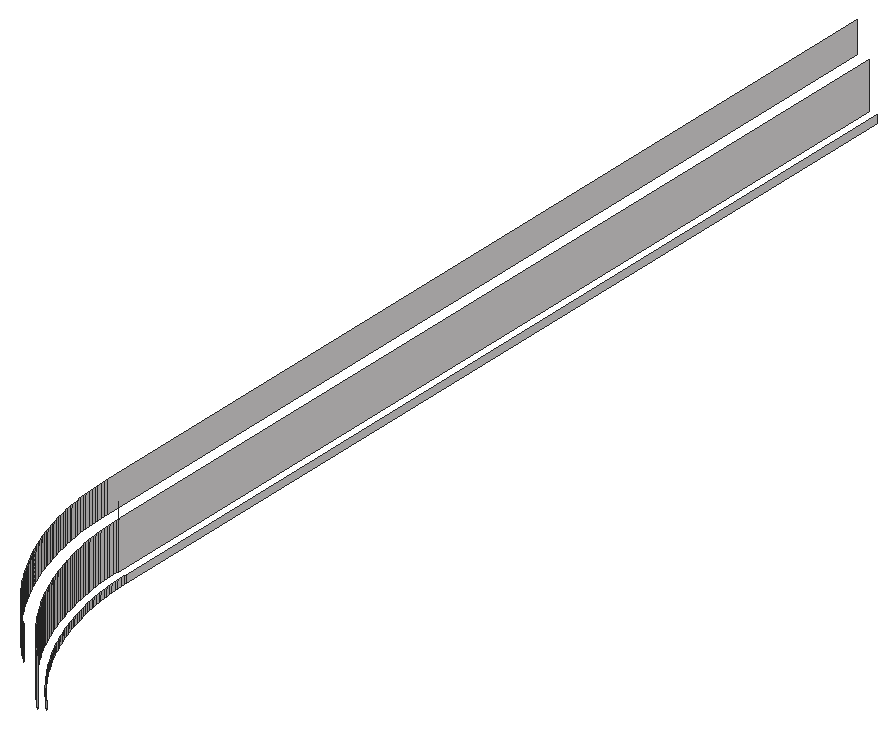
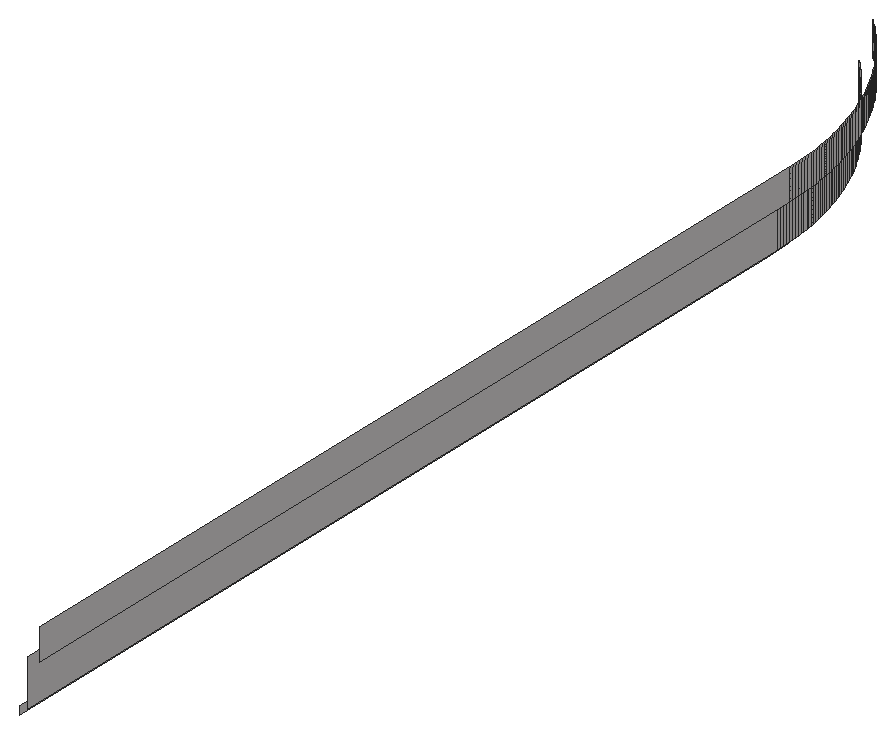
# SketchUp Ruby script. Lengths in inches.
U = 1.inch
M = Sketchup.active_model
def pt(a) = Geom::Point3d.new(a.map { |v| v * U })
def face(e, loops, mat)
  f = e.add_face(loops[0].map { |a| pt(a) })
  loops[1..].each { |l| e.add_face(l.map { |a| pt(a) }).erase! }
  f.material = f.back_material = mat if mat
  f
end
# faces: each face lists its corners as indices into pts; further lists are holes
def faces(e, pts, list, mat = nil) = list.each { |f| face(e, (f[0].is_a?(Array) ? f : [f]).map { |l| l.map { |i| pts[i] } }, mat) }
# xy, xz, yz: faces in a plane at the given z, y or x. An outline is a flat list of corners, or four numbers for a rectangle; further outlines are holes
def ring(l) = l.size == 4 ? [[l[0], l[1]], [l[2], l[1]], [l[2], l[3]], [l[0], l[3]]] : l.each_slice(2).to_a
def flat(e, list, mat, &to3) = list.each { |f| face(e, (f[0].is_a?(Array) ? f : [f]).map { |l| ring(l).map { |u, v| to3.(u, v) } }, mat) }
def xy(e, z, list, mat = nil) = flat(e, list, mat) { |x, y| [x, y, z] }
def xz(e, y, list, mat = nil) = flat(e, list, mat) { |x, z| [x, y, z] }
def yz(e, x, list, mat = nil) = flat(e, list, mat) { |y, z| [x, y, z] }
def lines(e, pts, list) = list.each { |a, b| e.add_line(pt(pts[a]), pt(pts[b])) }
# prism: a flat outline (further loops are holes) pulled along v
def prism(e, loops, v, mat = nil)
  f = face(e, loops, mat); d = Geom::Vector3d.new(v.map { |x| x * U })
  f.pushpull(f.normal.samedirection?(d) ? d.length : -d.length)
end
def box(e, o, s, mat = nil) = prism(e, [[o, [o[0] + s[0], o[1], o[2]], [o[0] + s[0], o[1] + s[1], o[2]], [o[0], o[1] + s[1], o[2]]]], [0, 0, s[2]], mat)
def at(x, y, z, deg = 0) = Geom::Transformation.translation(pt([x, y, z])) * Geom::Transformation.rotation(ORIGIN, Z_AXIS, deg.degrees)
def axes(o, x, y, z) = Geom::Transformation.new([*x, 0, *y, 0, *z, 0, *pt(o).to_a, 1])
def part(name) = M.definitions.add(name)
# library, detail: a bought-in or finely detailed component or shape, given as its bounding box
def library(name, o, s) = part(name).tap { |d| box(d.entities, o, s) }
def detail(e, o, s) = box(e.add_group.entities, o, s)
def put(e, d, t, mat = nil) = e.add_instance(d, t).tap { |i| i.material = mat if mat }
def group(e, t, mat = nil) = e.add_group.tap { |g| g.transformation = t; g.material = mat if mat }.entities
root = M.entities
M.materials.add("[Quartz Light Brown]").color = [215, 212, 212]
yz(root,185.5,[[320.18,493,320.7,497],[320.7,493,440.7,497]],"[Quartz Light Brown]")
yz(root,187,[[320.2,487,320.7,493],[320.7,487,440.7,493]],"[Quartz Light Brown]")
yz(root,188,[[320.22,486,320.7,487],[320.7,486,440.7,487]],"[Quartz Light Brown]")
p = [[197.5,295.94,486],[197.83,295.59,486],[197.83,295.59,487],[197.5,295.94,487],[197.18,296.31,486],[197.18,296.31,487],
  [196.86,296.67,486],[196.86,296.67,487],[196.55,297.04,486],[196.55,297.04,487],[196.25,297.42,486],[196.25,297.42,487],
  [195.94,297.79,486],[195.94,297.79,487],[195.65,298.18,486],[195.65,298.18,487],[195.35,298.5625,486],[195.35,298.5625,487],
  [195.07,298.95,486],[195.07,298.95,487],[194.78,299.35,486],[194.78,299.35,487],[194.51,299.74,486],[194.51,299.74,487],
  [194.24,300.14,486],[194.24,300.14,487],[193.97,300.55,486],[193.97,300.55,487],[193.71,300.96,486],[193.71,300.96,487],
  [193.45,301.37,486],[193.45,301.37,487],[193.2,301.78,486],[193.2,301.78,487],[192.96,302.2,486],[192.96,302.2,487],
  [192.72,302.62,486],[192.72,302.62,487],[192.48,303.05,486],[192.48,303.05,487],[192.26,303.47,486],[192.26,303.47,487],
  [192.03,303.9,486],[192.03,303.9,487],[191.82,304.34,486],[191.82,304.34,487],[191.6,304.77,486],[191.6,304.77,487],
  [191.4,305.21,486],[191.4,305.21,487],[191.2,305.65,486],[191.2,305.65,487],[191,306.1,486],[191,306.1,487],
  [190.82,306.54,486],[190.82,306.54,487],[190.63,306.99,486],[190.63,306.99,487],[190.46,307.44,486],[190.46,307.44,487],
  [190.29,307.89,486],[190.29,307.89,487],[190.12,308.35,486],[190.12,308.35,487],[189.96,308.81,486],[189.96,308.81,487],
  [189.8125,309.27,486],[189.8125,309.27,487],[189.66,309.73,486],[189.66,309.73,487],[189.52,310.19,486],[189.52,310.19,487],
  [189.39,310.66,486],[189.39,310.66,487],[189.26,311.125,486],[189.26,311.125,487],[189.14,311.59,486],[189.14,311.59,487],
  [189.02,312.0625,486],[189.02,312.0625,487],[188.91,312.54,486],[188.91,312.54,487],[188.81,313.01,486],[188.81,313.01,487],
  [188.71,313.48,486],[188.71,313.48,487],[188.62,313.96,486],[188.62,313.96,487],[188.53,314.44,486],[188.53,314.44,487],
  [188.46,314.91,486],[188.46,314.91,487],[188.38,315.39,486],[188.38,315.39,487],[188.32,315.87,486],[188.32,315.87,487],
  [188.26,316.35,486],[188.26,316.35,487],[188.2,316.83,486],[188.2,316.83,487],[188.16,317.32,486],[188.16,317.32,487],
  [188.11,317.8,486],[188.11,317.8,487],[188.08,318.28,486],[188.08,318.28,487],[188.05,318.76,486],[188.05,318.76,487],
  [188.03,319.25,486],[188.03,319.25,487],[188.01,319.73,486],[188.01,319.73,487],[188,320.22,486],[188,320.22,487],
  [198.13,293.83,487],[198.13,293.83,493],[197.78,294.18,493],[197.78,294.18,487],[197.4375,294.54,493],[197.4375,294.54,487],
  [197.1,294.91,493],[197.1,294.91,487],[196.76,295.27,493],[196.76,295.27,487],[196.43,295.65,493],[196.43,295.65,487],
  [196.1,296.02,493],[196.1,296.02,487],[195.78,296.4,493],[195.78,296.4,487],[195.47,296.79,493],[195.47,296.79,487],
  [195.16,297.18,493],[195.16,297.18,487],[194.85,297.57,493],[194.85,297.57,487],[194.55,297.96,493],[194.55,297.96,487],
  [194.26,298.37,493],[194.26,298.37,487],[193.97,298.77,493],[193.97,298.77,487],[193.68,299.18,493],[193.68,299.18,487],
  [193.4,299.59,493],[193.4,299.59,487],[193.13,300,493],[193.13,300,487],[192.86,300.42,493],[192.86,300.42,487],
  [192.6,300.85,493],[192.6,300.85,487],[192.34,301.27,493],[192.34,301.27,487],[192.09,301.7,493],[192.09,301.7,487],
  [191.85,302.13,493],[191.85,302.13,487],[191.6,302.57,493],[191.6,302.57,487],[191.37,303.01,493],[191.37,303.01,487],
  [191.14,303.45,493],[191.14,303.45,487],[190.92,303.89,493],[190.92,303.89,487],[190.7,304.34,493],[190.7,304.34,487],
  [190.49,304.79,493],[190.49,304.79,487],[190.29,305.25,493],[190.29,305.25,487],[190.09,305.7,493],[190.09,305.7,487],
  [189.89,306.16,493],[189.89,306.16,487],[189.71,306.62,493],[189.71,306.62,487],[189.52,307.08,493],[189.52,307.08,487],
  [189.35,307.55,493],[189.35,307.55,487],[189.18,308.02,493],[189.18,308.02,487],[189.02,308.49,493],[189.02,308.49,487],
  [188.86,308.96,493],[188.86,308.96,487],[188.71,309.43,493],[188.71,309.43,487],[188.56,309.91,493],[188.56,309.91,487],
  [188.43,310.39,493],[188.43,310.39,487],[188.29,310.87,493],[188.29,310.87,487],[188.17,311.35,493],[188.17,311.35,487],
  [188.05,311.83,493],[188.05,311.83,487],[187.9375,312.31,493],[187.9375,312.31,487],[187.83,312.8,493],[187.83,312.8,487],
  [187.73,313.29,493],[187.73,313.29,487],[187.64,313.78,493],[187.64,313.78,487],[187.55,314.27,493],[187.55,314.27,487],
  [187.47,314.76,493],[187.47,314.76,487],[187.39,315.25,493],[187.39,315.25,487],[187.33,315.74,493],[187.33,315.74,487],
  [187.26,316.23,493],[187.26,316.23,487],[187.21,316.73,493],[187.21,316.73,487],[187.16,317.22,493],[187.16,317.22,487],
  [187.12,317.72,493],[187.12,317.72,487],[187.08,318.22,493],[187.08,318.22,487],[187.05,318.71,493],[187.05,318.71,487],
  [187.03,319.21,493],[187.03,319.21,487],[187.01,319.71,493],[187.01,319.71,487],[187,320.2,493],[187,320.2,487],
  [197.4375,292.41,493],[197.81,292.05,493],[197.81,292.05,497],[197.4375,292.41,497],[197.07,292.77,493],[197.07,292.77,497],
  [196.71,293.14,493],[196.71,293.14,497],[196.35,293.51,493],[196.35,293.51,497],[195.99,293.89,493],[195.99,293.89,497],
  [195.65,294.27,493],[195.65,294.27,497],[195.3,294.66,493],[195.3,294.66,497],[194.96,295.05,493],[194.96,295.05,497],
  [194.63,295.44,493],[194.63,295.44,497],[194.3,295.84,493],[194.3,295.84,497],[193.98,296.25,493],[193.98,296.25,497],
  [193.66,296.65,493],[193.66,296.65,497],[193.35,297.07,493],[193.35,297.07,497],[193.04,297.48,493],[193.04,297.48,497],
  [192.74,297.9,493],[192.74,297.9,497],[192.45,298.33,493],[192.45,298.33,497],[192.16,298.76,493],[192.16,298.76,497],
  [191.87,299.1875,493],[191.87,299.1875,497],[191.59,299.625,493],[191.59,299.625,497],[191.32,300.0625,493],[191.32,300.0625,497],
  [191.05,300.5,493],[191.05,300.5,497],[190.79,300.95,493],[190.79,300.95,497],[190.54,301.4,493],[190.54,301.4,497],
  [190.29,301.85,493],[190.29,301.85,497],[190.04,302.31,493],[190.04,302.31,497],[189.81,302.77,493],[189.81,302.77,497],
  [189.57,303.23,493],[189.57,303.23,497],[189.35,303.7,493],[189.35,303.7,497],[189.13,304.16,493],[189.13,304.16,497],
  [188.91,304.63,493],[188.91,304.63,497],[188.71,305.11,493],[188.71,305.11,497],[188.51,305.59,493],[188.51,305.59,497],
  [188.3125,306.0625,493],[188.3125,306.0625,497],[188.125,306.55,493],[188.125,306.55,497],[187.94,307.03,493],[187.94,307.03,497],
  [187.77,307.52,493],[187.77,307.52,497],[187.6,308,493],[187.6,308,497],[187.43,308.49,493],[187.43,308.49,497],
  [187.28,308.99,493],[187.28,308.99,497],[187.125,309.48,493],[187.125,309.48,497],[186.98,309.98,493],[186.98,309.98,497],
  [186.85,310.48,493],[186.85,310.48,497],[186.72,310.98,493],[186.72,310.98,497],[186.59,311.48,493],[186.59,311.48,497],
  [186.47,311.98,493],[186.47,311.98,497],[186.36,312.49,493],[186.36,312.49,497],[186.26,312.99,493],[186.26,312.99,497],
  [186.16,313.5,493],[186.16,313.5,497],[186.07,314.01,493],[186.07,314.01,497],[185.99,314.52,493],[185.99,314.52,497],
  [185.91,315.03,493],[185.91,315.03,497],[185.84,315.55,493],[185.84,315.55,497],[185.77,316.06,493],[185.77,316.06,497],
  [185.72,316.57,493],[185.72,316.57,497],[185.67,317.09,493],[185.67,317.09,497],[185.62,317.6,493],[185.62,317.6,497],
  [185.58,318.12,493],[185.58,318.12,497],[185.55,318.63,493],[185.55,318.63,497],[185.53,319.15,493],[185.53,319.15,497],
  [185.51,319.67,493],[185.51,319.67,497],[185.5,320.18,493],[185.5,320.18,497],[187,320.7,493],[187,320.7,495]]
faces(root,p,[[0,1,2,3],[4,0,3,5],[6,4,5,7],[8,6,7,9],[10,8,9,11],[12,10,11,13],[14,12,13,15],[16,14,15,17],
  [18,16,17,19],[20,18,19,21],[22,20,21,23],[24,22,23,25],[26,24,25,27],[28,26,27,29],[30,28,29,31],[32,30,31,33],
  [34,32,33,35],[36,34,35,37],[38,36,37,39],[40,38,39,41],[42,40,41,43],[44,42,43,45],[46,44,45,47],[48,46,47,49],
  [50,48,49,51],[52,50,51,53],[54,52,53,55],[56,54,55,57],[58,56,57,59],[60,58,59,61],[62,60,61,63],[64,62,63,65],
  [66,64,65,67],[68,66,67,69],[70,68,69,71],[72,70,71,73],[74,72,73,75],[76,74,75,77],[78,76,77,79],[80,78,79,81],
  [82,80,81,83],[84,82,83,85],[86,84,85,87],[88,86,87,89],[90,88,89,91],[92,90,91,93],[94,92,93,95],[96,94,95,97],
  [98,96,97,99],[100,98,99,101],[102,100,101,103],[104,102,103,105],[106,104,105,107],[108,106,107,109],[110,108,109,111],[112,110,111,113],
  [114,115,116,117],[117,116,118,119],[119,118,120,121],[121,120,122,123],[123,122,124,125],[125,124,126,127],[127,126,128,129],[129,128,130,131],
  [131,130,132,133],[133,132,134,135],[135,134,136,137],[137,136,138,139],[139,138,140,141],[141,140,142,143],[143,142,144,145],[145,144,146,147],
  [147,146,148,149],[149,148,150,151],[151,150,152,153],[153,152,154,155],[155,154,156,157],[157,156,158,159],[159,158,160,161],[161,160,162,163],
  [163,162,164,165],[165,164,166,167],[167,166,168,169],[169,168,170,171],[171,170,172,173],[173,172,174,175],[175,174,176,177],[177,176,178,179],
  [179,178,180,181],[181,180,182,183],[183,182,184,185],[185,184,186,187],[187,186,188,189],[189,188,190,191],[191,190,192,193],[193,192,194,195],
  [195,194,196,197],[197,196,198,199],[199,198,200,201],[201,200,202,203],[203,202,204,205],[205,204,206,207],[207,206,208,209],[209,208,210,211],
  [211,210,212,213],[213,212,214,215],[215,214,216,217],[217,216,218,219],[219,218,220,221],[221,220,222,223],[223,222,224,225],[225,224,226,227],
  [227,226,228,229],[229,228,230,231],[231,230,232,233],[234,235,236,237],[238,234,237,239],[240,238,239,241],[242,240,241,243],[244,242,243,245],
  [246,244,245,247],[248,246,247,249],[250,248,249,251],[252,250,251,253],[254,252,253,255],[256,254,255,257],[258,256,257,259],[260,258,259,261],
  [262,260,261,263],[264,262,263,265],[266,264,265,267],[268,266,267,269],[270,268,269,271],[272,270,271,273],[274,272,273,275],[276,274,275,277],
  [278,276,277,279],[280,278,279,281],[282,280,281,283],[284,282,283,285],[286,284,285,287],[288,286,287,289],[290,288,289,291],[292,290,291,293],
  [294,292,293,295],[296,294,295,297],[298,296,297,299],[300,298,299,301],[302,300,301,303],[304,302,303,305],[306,304,305,307],[308,306,307,309],
  [310,308,309,311],[312,310,311,313],[314,312,313,315],[316,314,315,317],[318,316,317,319],[320,318,319,321],[322,320,321,323],[324,322,323,325],
  [326,324,325,327],[328,326,327,329],[330,328,329,331],[332,330,331,333],[334,332,333,335],[336,334,335,337],[338,336,337,339],[340,338,339,341],
  [342,340,341,343],[344,342,343,345],[346,344,345,347],[348,346,347,349],[350,348,349,351],[352,350,351,353],[354,352,353,355],[356,354,355,357]],"[Quartz Light Brown]")
lines(root,p,[[358,359]])
